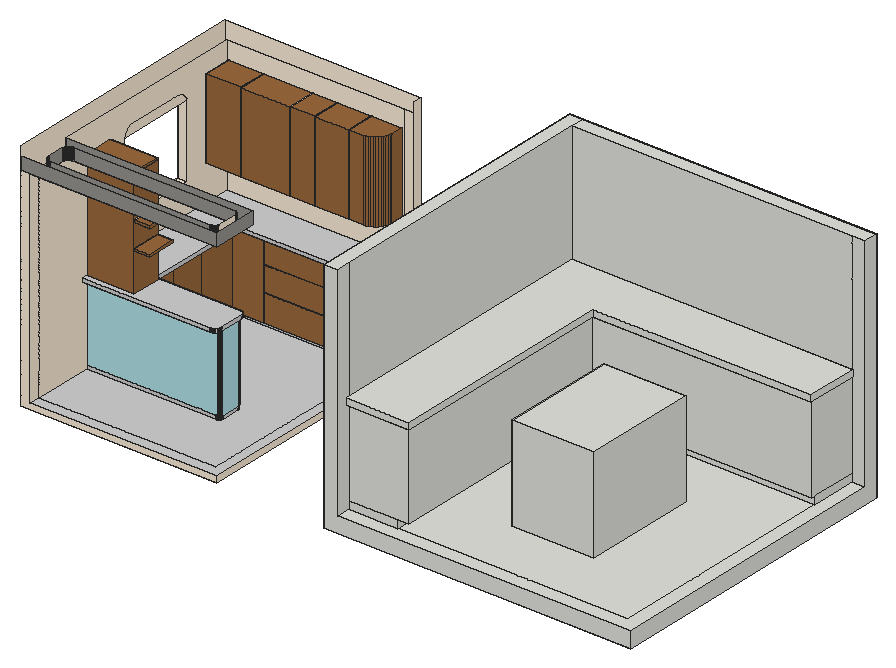
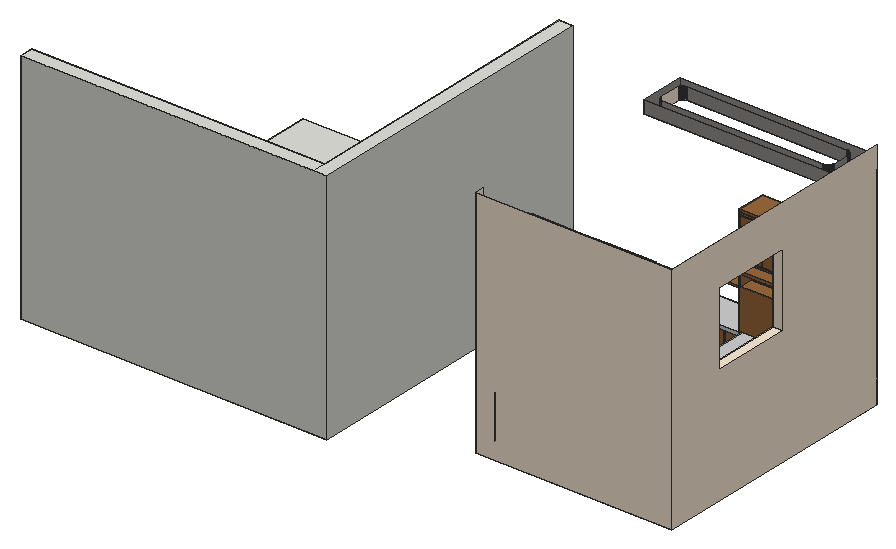
# SketchUp Ruby script. Lengths in inches.
U = 1.inch
M = Sketchup.active_model
def pt(a) = Geom::Point3d.new(a.map { |v| v * U })
def face(e, loops, mat)
  f = e.add_face(loops[0].map { |a| pt(a) })
  loops[1..].each { |l| e.add_face(l.map { |a| pt(a) }).erase! }
  f.material = f.back_material = mat if mat
  f
end
# faces: each face lists its corners as indices into pts; further lists are holes
def faces(e, pts, list, mat = nil) = list.each { |f| face(e, (f[0].is_a?(Array) ? f : [f]).map { |l| l.map { |i| pts[i] } }, mat) }
# xy, xz, yz: faces in a plane at the given z, y or x. An outline is a flat list of corners, or four numbers for a rectangle; further outlines are holes
def ring(l) = l.size == 4 ? [[l[0], l[1]], [l[2], l[1]], [l[2], l[3]], [l[0], l[3]]] : l.each_slice(2).to_a
def flat(e, list, mat, &to3) = list.each { |f| face(e, (f[0].is_a?(Array) ? f : [f]).map { |l| ring(l).map { |u, v| to3.(u, v) } }, mat) }
def xy(e, z, list, mat = nil) = flat(e, list, mat) { |x, y| [x, y, z] }
def xz(e, y, list, mat = nil) = flat(e, list, mat) { |x, z| [x, y, z] }
def yz(e, x, list, mat = nil) = flat(e, list, mat) { |y, z| [x, y, z] }
def lines(e, pts, list) = list.each { |a, b| e.add_line(pt(pts[a]), pt(pts[b])) }
# prism: a flat outline (further loops are holes) pulled along v
def prism(e, loops, v, mat = nil)
  f = face(e, loops, mat); d = Geom::Vector3d.new(v.map { |x| x * U })
  f.pushpull(f.normal.samedirection?(d) ? d.length : -d.length)
end
def box(e, o, s, mat = nil) = prism(e, [[o, [o[0] + s[0], o[1], o[2]], [o[0] + s[0], o[1] + s[1], o[2]], [o[0], o[1] + s[1], o[2]]]], [0, 0, s[2]], mat)
def at(x, y, z, deg = 0) = Geom::Transformation.translation(pt([x, y, z])) * Geom::Transformation.rotation(ORIGIN, Z_AXIS, deg.degrees)
def axes(o, x, y, z) = Geom::Transformation.new([*x, 0, *y, 0, *z, 0, *pt(o).to_a, 1])
def part(name) = M.definitions.add(name)
# library, detail: a bought-in or finely detailed component or shape, given as its bounding box
def library(name, o, s) = part(name).tap { |d| box(d.entities, o, s) }
def detail(e, o, s) = box(e.add_group.entities, o, s)
def put(e, d, t, mat = nil) = e.add_instance(d, t).tap { |i| i.material = mat if mat }
def group(e, t, mat = nil) = e.add_group.tap { |g| g.transformation = t; g.material = mat if mat }.entities
root = M.entities
M.materials.add("[0028_AntiqueWhite]").color = [250, 235, 215]
M.materials.add("[0094_PowderBlue]").color = [176, 224, 230]
M.materials.add("[0095_LightBlue]").color = [173, 216, 230]
M.materials.add("[Carrera Marble]").color = [207, 207, 207]
M.materials.add("[Granite Light Gray]").color = [149, 148, 144]
M.materials.add("[Wood Floor]").color = [155, 105, 61]
xy(root,0,[[313.34,0,630.34,317]])
xy(root,3.27,[[0,0,203.125,263.6875]],"[0028_AntiqueWhite]")
xy(root,9.21,[[10.23,0,203.125,0,203.125,253.46,188.43,253.46,189.04,253.33,189.625,253.14,190.1875,252.87,190.71,252.54,191.19,252.15,191.625,251.71,192,251.22,192.32,250.6875,192.57,250.12,192.75,249.53,192.86,248.92,192.89,248.3,192.89,11.5625,10.23,11.5625],[10.23,11.5625,192.89,11.5625,192.89,223.31,192.85,222.61,192.71,221.92,192.49,221.26,192.18,220.63,191.79,220.05,191.32,219.52,190.8,219.06,190.21,218.67,189.59,218.36,188.92,218.13,188.23,218,187.53,217.95,44.21,217.95,44.21,99.7,144.02,99.7,144.6,99.66,145.16,99.55,145.7,99.37,146.21,99.11,146.6875,98.8,147.12,98.42,147.49,97.99,147.8125,97.51,148.07,97,148.25,96.46,148.36,95.9,148.4,95.33,148.4,76.65,148.29,76.11,148.11,75.59,147.875,75.09,147.58,74.63,147.23,74.2,146.84,73.82,146.4,73.49,145.93,73.21,145.43,72.99,144.91,72.83,144.37,72.73,143.82,72.7,10.23,72.7]],"[Carrera Marble]")
xy(root,13.4,[[44.71,99.7,44.71,101.2,47.02,101.2,47.02,102.89,74.24,102.89,74.24,99.7],[74.74,99.7,110.3,102.89],[110.8,99.7,144.3,102.89],[44.21,101.2,44.21,138.64,47.02,138.64,47.02,102.89,44.71,102.89,44.71,101.2],[44.71,101.2,47.02,102.89],
  [44.21,139.14,47.02,174.76],[44.21,175.26,44.21,216.45,45.71,216.45,45.71,214.45,47.02,214.45,47.02,175.26],[45.71,214.45,47.02,216.45],[47.02,214.45,47.02,216.45,45.71,216.45,45.71,217.95,79.77,217.95,79.77,214.45],[80.27,214.45,151.02,217.95],
  [151.52,214.45,187.8,217.95]],"[0028_AntiqueWhite]")
xy(root,16.1875,[[327.62,0,630.34,0,630.34,302.72,616.07,302.72,616.07,14.28,327.62,14.28],[378.34,14.28,616.07,255.04]])
xy(root,23.9375,[[378.34,14.28,378.34,256.85,400.15,256.85,400.15,251.16,389.53,251.16,389.53,14.28],[400.15,251.16,400.15,256.85,378.34,256.85,378.34,302.72,616.07,302.72,616.07,251.16]])
xy(root,41.65,[[80.27,214.45,151.02,217.95]],"[0028_AntiqueWhite]")
xy(root,42.15,[[80.27,214.45,151.02,217.95]],"[0028_AntiqueWhite]")
xy(root,67.84,[[80.27,214.45,151.02,217.95]],"[Wood Floor]")
xy(root,68.34,[[80.27,214.45,151.02,217.95]],"[Wood Floor]")
xy(root,91.52,[[44.71,99.7,74.24,99.7,74.24,102.89,47.02,102.89,47.02,101.2,44.71,101.2],[74.74,99.7,110.3,102.89],[110.8,99.7,144.3,102.89],[44.21,101.2,44.71,101.2,44.71,102.89,47.02,102.89,47.02,138.64,44.21,138.64],[44.71,101.2,47.02,102.89],
  [44.21,139.14,47.02,174.76],[44.21,175.26,47.02,175.26,47.02,214.45,45.71,214.45,45.71,216.45,44.21,216.45],[45.71,214.45,47.02,216.45],[47.02,214.45,79.77,214.45,79.77,217.95,45.71,217.95,45.71,216.45,47.02,216.45],[80.27,214.45,151.02,217.95],
  [151.52,214.45,187.8,217.95]],"[0028_AntiqueWhite]")
xy(root,92.02,[[10.23,67.2,10.23,253.46,192.89,253.46,192.89,221.5,192.8125,220.24,192.5625,219,192.16,217.8,191.6,216.66,190.89,215.61,190.06,214.66,189.11,213.82,188.06,213.12,186.92,212.5625,185.72,212.15,184.48,211.91,183.22,211.82,56.15,211.82,56.15,105.01,142.61,105.01,143.36,104.97,144.11,104.83,144.83,104.61,145.53,104.31,146.18,103.92,146.78,103.47,147.32,102.9375,147.8,102.35,148.21,101.71,148.53,101.03,148.78,100.3125,148.93,99.57,148.93,74.1875,148.875,73.27,148.7,72.38,148.4,71.51,148,70.69,147.49,69.93,146.89,69.25,146.2,68.64,145.44,68.14,144.62,67.73,143.75,67.4375,142.86,67.26,141.95,67.2]],"[0028_AntiqueWhite]")
xy(root,95.52,[[10.23,67.2,141.95,67.2,142.86,67.26,143.75,67.4375,144.62,67.73,145.44,68.14,146.2,68.64,146.89,69.25,147.49,69.93,148,70.69,148.4,71.51,148.7,72.38,148.875,73.27,148.93,74.1875,148.93,99.57,148.78,100.3125,148.53,101.03,148.21,101.71,147.8,102.35,147.32,102.9375,146.78,103.47,146.18,103.92,145.53,104.31,144.83,104.61,144.11,104.83,143.36,104.97,142.61,105.01,56.15,105.01,56.15,211.82,183.22,211.82,184.48,211.91,185.72,212.15,186.92,212.5625,188.06,213.12,189.11,213.82,190.06,214.66,190.89,215.61,191.6,216.66,192.16,217.8,192.5625,219,192.8125,220.24,192.89,221.5,192.89,253.46,10.23,253.46,10.23,102.82,59.29,102.82,59.29,72.57,10.23,72.57]],"[Carrera Marble]")
xy(root,114.0625,[[327.62,10.96,392.71,14.28],[389.53,14.28,392.71,248.66],[389.53,248.66,617.63,302.72]])
xy(root,120.6875,[[327.62,10.96,392.71,10.96,392.71,248.66,617.63,248.66,617.63,302.72,327.62,302.72]])
xy(root,124.52,[[0,120.375,10.23,202.75]],"[0028_AntiqueWhite]")
xy(root,133.59,[[12.23,224.21,48.23,253.46],[48.73,224.21,98.92,253.46],[99.42,224.21,124.36,253.46],[124.86,224.21,159.42,253.46],[159.92,224.21,159.92,253.46,190.89,253.46,190.89,241.28,190.8,239.6875,190.76,239.17,190.38,237.11,189.74,235.1,188.87,233.19,187.76,231.39,186.44,229.75,184.9375,228.28,183.26,227.01,181.44,225.95,179.51,225.12,177.48,224.54,175.41,224.21]],"[Wood Floor]")
xy(root,135.54,[[59.29,72.57,75.67,102.82]],"[Wood Floor]")
xy(root,137.54,[[59.29,72.57,75.67,102.82],[12.23,89.76,57.29,102.82]],"[Wood Floor]")
xy(root,148.79,[[12.23,89.76,57.29,102.82]],"[Wood Floor]")
xy(root,150.79,[[12.23,89.76,57.29,102.82]],"[Wood Floor]")
xy(root,161.85,[[59.29,72.57,75.67,102.82],[12.23,89.76,57.29,102.82]],"[Wood Floor]")
xy(root,163.85,[[59.29,72.57,75.67,102.82]],"[Wood Floor]")
xy(root,164.15,[[12.23,102.82,34.61,104.76],[34.81,102.82,57.29,104.76]],"[Wood Floor]")
xy(root,200.46,[[0,120.375,10.23,202.75]],"[0028_AntiqueWhite]")
xy(root,203.84,[[12.23,102.82,34.61,104.76],[34.81,102.82,57.29,104.76]],"[Wood Floor]")
xy(root,205.84,[[10.23,72.26,59.67,72.57],[59.29,72.57,59.67,103.14],[10.23,102.82,59.29,103.14]],"[0028_AntiqueWhite]")
xy(root,206.27,[[10.23,72.26,59.67,72.57],[59.29,72.57,59.67,103.14],[10.23,102.82,59.29,103.14]],"[Wood Floor]")
xy(root,208.27,[[10.23,72.57,59.29,102.82]],"[Wood Floor]")
xy(root,216.15,[[12.23,224.21,48.23,253.46],[48.73,224.21,98.92,253.46],[99.42,224.21,124.36,253.46],[124.86,224.21,159.42,253.46],[159.92,224.21,175.41,224.21,177.48,224.54,179.51,225.12,181.44,225.95,183.26,227.01,184.9375,228.28,186.44,229.75,187.76,231.39,188.87,233.19,189.74,235.1,190.38,237.11,190.76,239.17,190.89,241.28,190.89,253.46,159.92,253.46]],"[Wood Floor]")
xy(root,221.34,[[[10.23,0,203.125,45.92],[24.97,7.66,190.05,7.66,190.7,7.7,191.34,7.8125,191.97,8,192.5625,8.27,193.125,8.6,193.64,9,194.11,9.46,194.52,9.97,194.86,10.52,195.14,11.11,195.34,11.73,195.47,12.37,195.47,33.28,195.35,33.9,195.16,34.5,194.92,35.08,194.61,35.63,194.24,36.14,193.82,36.61,193.35,37.03,192.84,37.4,192.29,37.71,191.71,37.96,191.11,38.14,190.49,38.26,24.48,38.26,23.62,38.21,22.77,38.04,21.95,37.76,21.18,37.38,20.47,36.9,19.82,36.33,19.25,35.69,18.77,34.97,18.39,34.2,18.11,33.38,17.94,32.53,17.89,31.67,17.89,14.74,17.95,13.82,18.13,12.91,18.43,12.03,18.84,11.2,19.35,10.43,19.96,9.73,20.66,9.12,21.43,8.61,22.26,8.2,23.14,7.9,24.05,7.72]]],"[Granite Light Gray]")
xy(root,243.9,[[313.34,0,327.62,317],[327.62,302.72,630.34,317]])
xz(root,0,[[313.34,0,630.34,0,630.34,16.1875,327.62,16.1875,327.62,243.9,313.34,243.9]])
xz(root,0,[[0,3.27,203.125,3.27,203.125,9.21,10.23,9.21,10.23,221.34,0,221.34]],"[0028_AntiqueWhite]")
xz(root,0,[[0,221.34,203.125,234.21]],"[Granite Light Gray]")
xz(root,7.66,[[24.97,221.34,190.05,233.77]],"[Granite Light Gray]")
xz(root,10.96,[[327.62,114.0625,392.71,120.6875]])
xz(root,38.26,[[24.48,221.34,190.49,233.77]],"[Granite Light Gray]")
xz(root,45.92,[[10.23,221.34,203.125,234.21]],"[Granite Light Gray]")
xz(root,67.2,[[10.23,92.02,141.95,95.52]],"[Carrera Marble]")
xz(root,72.26,[[10.23,205.84,59.67,206.27]],"[Wood Floor]")
xz(root,72.57,[[10.23,95.52,59.29,205.84],[59.29,135.54,75.67,137.54],[59.29,161.85,75.67,163.85],[10.23,206.27,59.29,208.27]],"[Wood Floor]")
xz(root,89.76,[[12.23,137.54,57.29,148.79],[12.23,150.79,57.29,161.85]],"[Wood Floor]")
xz(root,99.7,[[44.21,9.21,144.02,12.9],[44.71,13.4,74.24,91.52],[74.74,13.4,110.3,91.52],[110.8,13.4,144.3,91.52]],"[0028_AntiqueWhite]")
xz(root,101.2,[[44.21,13.4,47.02,91.52]],"[0028_AntiqueWhite]")
xz(root,102.82,[[[10.23,95.52,59.29,205.84],[34.81,164.15,57.29,203.84],[12.23,164.15,34.61,203.84],[12.23,137.54,57.29,148.79],[12.23,150.79,57.29,161.85]],[59.29,135.54,75.67,137.54],[59.29,161.85,75.67,163.85],[10.23,206.27,59.29,208.27]],"[Wood Floor]")
xz(root,102.89,[[44.71,13.4,74.24,91.52],[74.74,13.4,110.3,91.52],[110.8,13.4,144.3,91.52]],"[Wood Floor]")
xz(root,103.14,[[10.23,205.84,59.67,206.27]],"[Wood Floor]")
xz(root,104.76,[[12.23,164.15,34.61,203.84],[34.81,164.15,57.29,203.84]],"[Wood Floor]")
xz(root,105.01,[[56.15,92.02,142.61,95.52]],"[Carrera Marble]")
xz(root,120.375,[[0,124.52,10.23,200.46]],"[0028_AntiqueWhite]")
xz(root,138.64,[[44.21,13.4,47.02,91.52]],"[Wood Floor]")
xz(root,139.14,[[44.21,13.4,47.02,91.52]],"[Wood Floor]")
xz(root,174.76,[[44.21,13.4,47.02,91.52]],"[Wood Floor]")
xz(root,175.26,[[44.21,13.4,47.02,91.52]],"[Wood Floor]")
xz(root,202.75,[[0,124.52,10.23,200.46]],"[0028_AntiqueWhite]")
xz(root,211.82,[[56.15,92.02,183.22,95.52]],"[Carrera Marble]")
xz(root,214.45,[[45.71,13.4,79.77,91.52],[80.27,13.4,151.02,41.65],[151.52,13.4,187.8,91.52],[80.27,42.15,151.02,67.84],[80.27,68.34,151.02,91.52]],"[Wood Floor]")
xz(root,216.45,[[44.21,13.4,47.02,91.52]],"[0028_AntiqueWhite]")
xz(root,217.95,[[45.71,13.4,79.77,91.52],[80.27,13.4,151.02,41.65],[151.52,13.4,187.8,91.52],[80.27,42.15,151.02,67.84],[80.27,68.34,151.02,91.52]],"[0028_AntiqueWhite]")
xz(root,224.21,[[12.23,133.59,48.23,216.15],[48.73,133.59,98.92,216.15],[99.42,133.59,124.36,216.15],[124.86,133.59,159.42,216.15],[159.92,133.59,175.41,216.15]],"[Wood Floor]")
xz(root,248.66,[[392.71,114.0625,617.63,120.6875]])
xz(root,253.46,[[188.43,9.21,192.89,12.9],[192.89,9.21,203.125,234.21],[189.47,12.9,192.89,92.02],[[10.23,95.52,192.89,234.21],[48.73,133.59,98.92,216.15],[12.23,133.59,48.23,216.15],[124.86,133.59,159.42,216.15],[159.92,133.59,190.89,216.15],[99.42,133.59,124.36,216.15]]],"[0028_AntiqueWhite]")
xz(root,263.6875,[[0,3.27,203.125,243.9]],"[0028_AntiqueWhite]")
xz(root,302.72,[[616.07,16.1875,630.34,16.1875,630.34,243.9,616.07,243.9,616.07,120.6875,617.63,120.6875,617.63,114.0625,616.07,114.0625],[327.62,120.6875,616.07,243.9]])
xz(root,317,[[313.34,0,630.34,243.9]])
yz(root,0,[[[0,3.27,263.6875,243.9],[120.375,124.52,202.75,200.46]]],"[0028_AntiqueWhite]")
yz(root,10.23,[[0,9.21,11.5625,221.34],[[11.5625,9.21,72.7,9.21,72.7,92.02,67.2,92.02,67.2,95.52,72.57,95.52,72.57,205.84,72.26,205.84,72.26,206.27,72.57,206.27,72.57,208.27,102.82,208.27,102.82,206.27,103.14,206.27,103.14,205.84,102.82,205.84,102.82,95.52,253.46,95.52,253.46,234.21,45.92,234.21,45.92,221.34,11.5625,221.34],[120.375,124.52,120.375,200.46,120.84,201.84,121.46,203.17,122.21,204.42,123.09,205.58,124.1,206.64,125.21,207.59,126.42,208.41,127.71,209.09,129.07,209.63,130.47,210.02,131.92,210.26,133.375,210.34,189.75,210.34,191.21,210.26,192.65,210.02,194.06,209.63,195.41,209.09,196.7,208.41,197.91,207.59,199.03,206.64,200.03,205.58,200.91,204.42,201.67,203.17,202.28,201.84,202.75,200.46,202.75,124.52]],[120.375,200.46,202.75,200.46,202.28,201.84,201.67,203.17,200.91,204.42,200.03,205.58,199.03,206.64,197.91,207.59,196.7,208.41,195.41,209.09,194.06,209.63,192.65,210.02,191.21,210.26,189.75,210.34,133.375,210.34,131.92,210.26,130.47,210.02,129.07,209.63,127.71,209.09,126.42,208.41,125.21,207.59,124.1,206.64,123.09,205.58,122.21,204.42,121.46,203.17,120.84,201.84]],"[0028_AntiqueWhite]")
yz(root,12.23,[[102.82,164.15,104.76,203.84]],"[0028_AntiqueWhite]")
yz(root,12.23,[[224.21,133.59,253.46,216.15],[89.76,137.54,102.82,148.79],[89.76,150.79,102.82,161.85]],"[Wood Floor]")
yz(root,17.89,[[14.74,221.34,31.67,233.77]],"[Granite Light Gray]")
yz(root,34.61,[[102.82,164.15,104.76,203.84]],"[Wood Floor]")
yz(root,34.81,[[102.82,164.15,104.76,203.84]],"[0028_AntiqueWhite]")
yz(root,44.21,[[101.2,13.4,138.64,91.52],[139.14,13.4,174.76,91.52],[175.26,13.4,216.45,91.52]],"[0028_AntiqueWhite]")
yz(root,44.71,[[99.7,13.4,102.89,91.52]],"[0028_AntiqueWhite]")
yz(root,45.71,[[214.45,13.4,217.95,91.52]],"[0028_AntiqueWhite]")
yz(root,47.02,[[101.2,13.4,138.64,91.52],[139.14,13.4,174.76,91.52],[175.26,13.4,216.45,91.52]],"[Wood Floor]")
yz(root,48.23,[[224.21,133.59,253.46,216.15]],"[0028_AntiqueWhite]")
yz(root,48.73,[[224.21,133.59,253.46,216.15]],"[0028_AntiqueWhite]")
yz(root,56.15,[[105.01,92.02,211.82,95.52]],"[Carrera Marble]")
yz(root,57.29,[[89.76,137.54,102.82,148.79],[89.76,150.79,102.82,161.85],[102.82,164.15,104.76,203.84]],"[Wood Floor]")
yz(root,59.29,[[72.57,135.54,102.82,137.54],[72.57,161.85,102.82,163.85]],"[0028_AntiqueWhite]")
yz(root,59.29,[[72.57,95.52,102.82,135.54],[72.57,137.54,102.82,161.85],[72.57,163.85,102.82,205.84],[72.57,206.27,102.82,208.27]],"[Wood Floor]")
yz(root,59.67,[[72.26,205.84,103.14,206.27]],"[Wood Floor]")
yz(root,74.24,[[99.7,13.4,102.89,91.52]],"[0028_AntiqueWhite]")
yz(root,74.74,[[99.7,13.4,102.89,91.52]],"[0028_AntiqueWhite]")
yz(root,75.67,[[72.57,135.54,102.82,137.54],[72.57,161.85,102.82,163.85]],"[Wood Floor]")
yz(root,79.77,[[214.45,13.4,217.95,91.52]],"[0028_AntiqueWhite]")
yz(root,80.27,[[214.45,13.4,217.95,41.65],[214.45,42.15,217.95,67.84],[214.45,68.34,217.95,91.52]],"[0028_AntiqueWhite]")
yz(root,98.92,[[224.21,133.59,253.46,216.15]],"[0028_AntiqueWhite]")
yz(root,99.42,[[224.21,133.59,253.46,216.15]],"[0028_AntiqueWhite]")
yz(root,110.3,[[99.7,13.4,102.89,91.52]],"[0028_AntiqueWhite]")
yz(root,110.8,[[99.7,13.4,102.89,91.52]],"[0028_AntiqueWhite]")
yz(root,124.36,[[224.21,133.59,253.46,216.15]],"[0028_AntiqueWhite]")
yz(root,124.86,[[224.21,133.59,253.46,216.15]],"[0028_AntiqueWhite]")
yz(root,144.3,[[99.7,13.4,102.89,91.52]],"[Wood Floor]")
yz(root,148.93,[[74.1875,92.02,99.57,95.52]],"[Carrera Marble]")
yz(root,151.02,[[214.45,13.4,217.95,41.65]],"[0028_AntiqueWhite]")
yz(root,151.02,[[214.45,42.15,217.95,67.84],[214.45,68.34,217.95,91.52]],"[Wood Floor]")
yz(root,151.52,[[214.45,13.4,217.95,91.52]],"[0028_AntiqueWhite]")
yz(root,159.42,[[224.21,133.59,253.46,216.15]],"[0028_AntiqueWhite]")
yz(root,159.92,[[224.21,133.59,253.46,216.15]],"[0028_AntiqueWhite]")
yz(root,187.8,[[214.45,13.4,217.95,91.52]],"[Wood Floor]")
yz(root,190.89,[[241.28,133.59,253.46,216.15]],"[Wood Floor]")
yz(root,192.89,[[221.5,92.02,253.46,95.52]],"[Carrera Marble]")
yz(root,195.47,[[12.37,221.34,33.28,233.77]],"[0028_AntiqueWhite]")
yz(root,203.125,[[0,3.27,263.6875,3.27,263.6875,243.9,253.46,243.9,253.46,9.21,0,9.21]],"[0028_AntiqueWhite]")
yz(root,203.125,[[0,221.34,45.92,234.21]],"[Granite Light Gray]")
yz(root,313.34,[[0,0,317,243.9]])
yz(root,327.62,[[0,16.1875,14.28,16.1875,14.28,114.0625,10.96,114.0625,10.96,120.6875,14.28,120.6875,14.28,243.9,0,243.9],[14.28,120.6875,302.72,243.9]])
yz(root,392.71,[[10.96,114.0625,248.66,120.6875]])
yz(root,617.63,[[248.66,114.0625,302.72,120.6875]])
yz(root,630.34,[[0,0,317,0,317,243.9,302.72,243.9,302.72,16.1875,0,16.1875]])
p = [[142.86,67.26,95.52],[141.95,67.2,95.52],[141.95,67.2,92.02],[142.86,67.26,92.02],[143.75,67.4375,95.52],[143.75,67.4375,92.02],
  [144.62,67.73,95.52],[144.62,67.73,92.02],[145.44,68.14,95.52],[145.44,68.14,92.02],[146.2,68.64,95.52],[146.2,68.64,92.02],
  [146.89,69.25,95.52],[146.89,69.25,92.02],[147.49,69.93,95.52],[147.49,69.93,92.02],[148,70.69,95.52],[148,70.69,92.02],
  [148.4,71.51,95.52],[148.4,71.51,92.02],[148.7,72.38,95.52],[148.7,72.38,92.02],[148.875,73.27,95.52],[148.875,73.27,92.02],
  [148.93,74.1875,95.52],[148.93,74.1875,92.02],[148.78,100.3125,95.52],[148.93,99.57,95.52],[148.93,99.57,92.02],[148.78,100.3125,92.02],
  [148.53,101.03,95.52],[148.53,101.03,92.02],[148.21,101.71,95.52],[148.21,101.71,92.02],[147.8,102.35,95.52],[147.8,102.35,92.02],
  [147.32,102.9375,95.52],[147.32,102.9375,92.02],[146.78,103.47,95.52],[146.78,103.47,92.02],[146.18,103.92,95.52],[146.18,103.92,92.02],
  [145.53,104.31,95.52],[145.53,104.31,92.02],[144.83,104.61,95.52],[144.83,104.61,92.02],[144.11,104.83,95.52],[144.11,104.83,92.02],
  [143.36,104.97,95.52],[143.36,104.97,92.02],[142.61,105.01,95.52],[142.61,105.01,92.02],[184.48,211.91,95.52],[183.22,211.82,95.52],
  [183.22,211.82,92.02],[184.48,211.91,92.02],[185.72,212.15,95.52],[185.72,212.15,92.02],[186.92,212.5625,95.52],[186.92,212.5625,92.02],
  [188.06,213.12,95.52],[188.06,213.12,92.02],[189.11,213.82,95.52],[189.11,213.82,92.02],[190.06,214.66,95.52],[190.06,214.66,92.02],
  [190.89,215.61,95.52],[190.89,215.61,92.02],[191.6,216.66,95.52],[191.6,216.66,92.02],[192.16,217.8,95.52],[192.16,217.8,92.02],
  [192.5625,219,95.52],[192.5625,219,92.02],[192.8125,220.24,95.52],[192.8125,220.24,92.02],[192.89,221.5,95.52],[192.89,221.5,92.02],
  [177.48,224.54,216.15],[175.41,224.21,216.15],[175.41,224.21,133.59],[177.48,224.54,133.59],[179.51,225.12,216.15],[179.51,225.12,133.59],
  [181.44,225.95,216.15],[181.44,225.95,133.59],[183.26,227.01,216.15],[183.26,227.01,133.59],[184.9375,228.28,216.15],[184.9375,228.28,133.59],
  [186.44,229.75,216.15],[186.44,229.75,133.59],[187.76,231.39,216.15],[187.76,231.39,133.59],[188.87,233.19,216.15],[188.87,233.19,133.59],
  [189.74,235.1,216.15],[189.74,235.1,133.59],[190.38,237.11,216.15],[190.38,237.11,133.59],[190.76,239.17,216.15],[190.76,239.17,133.59],
  [190.89,241.28,216.15],[190.8,239.6875,133.59],[190.89,241.28,133.59],[24.05,7.72,221.34],[23.14,7.9,221.34],[23.14,7.9,233.77],
  [24.05,7.72,233.77],[24.97,7.66,221.34],[24.97,7.66,233.77],[190.7,7.7,221.34],[190.05,7.66,221.34],[190.05,7.66,233.77],
  [190.7,7.7,233.77],[191.34,7.8125,221.34],[191.34,7.8125,233.77],[191.97,8,221.34],[191.97,8,233.77],[22.26,8.2,221.34],
  [22.26,8.2,233.77],[192.5625,8.27,221.34],[192.5625,8.27,233.77],[21.43,8.61,221.34],[21.43,8.61,233.77],[193.125,8.6,221.34],
  [193.125,8.6,233.77],[20.66,9.12,221.34],[20.66,9.12,233.77],[193.64,9,221.34],[193.64,9,233.77],[194.11,9.46,221.34],
  [194.11,9.46,233.77],[19.96,9.73,221.34],[19.96,9.73,233.77],[194.52,9.97,221.34],[194.52,9.97,233.77],[19.35,10.43,221.34],
  [19.35,10.43,233.77],[194.86,10.52,221.34],[194.86,10.52,233.77],[18.84,11.2,221.34],[18.84,11.2,233.77],[195.14,11.11,221.34],
  [195.14,11.11,233.77],[195.34,11.73,221.34],[195.34,11.73,233.77],[18.43,12.03,221.34],[18.43,12.03,233.77],[195.47,12.37,221.34],
  [195.47,12.37,233.77],[18.13,12.91,221.34],[18.13,12.91,233.77],[17.95,13.82,221.34],[17.95,13.82,233.77],[17.89,14.74,221.34],
  [17.89,14.74,233.77],[17.89,31.67,221.34],[17.94,32.53,221.34],[17.94,32.53,233.77],[17.89,31.67,233.77],[18.11,33.38,221.34],
  [18.11,33.38,233.77],[195.35,33.9,221.34],[195.47,33.28,221.34],[195.47,33.28,233.77],[195.35,33.9,233.77],[18.39,34.2,221.34],
  [18.39,34.2,233.77],[195.16,34.5,221.34],[195.16,34.5,233.77],[18.77,34.97,221.34],[18.77,34.97,233.77],[194.92,35.08,221.34],
  [194.92,35.08,233.77],[19.25,35.69,221.34],[19.25,35.69,233.77],[194.61,35.63,221.34],[194.61,35.63,233.77],[194.24,36.14,221.34],
  [194.24,36.14,233.77],[19.82,36.33,221.34],[19.82,36.33,233.77],[193.82,36.61,221.34],[193.82,36.61,233.77],[20.47,36.9,221.34],
  [20.47,36.9,233.77],[193.35,37.03,221.34],[193.35,37.03,233.77],[21.18,37.38,221.34],[21.18,37.38,233.77],[192.84,37.4,221.34],
  [192.84,37.4,233.77],[21.95,37.76,221.34],[21.95,37.76,233.77],[192.29,37.71,221.34],[192.29,37.71,233.77],[191.71,37.96,221.34],
  [191.71,37.96,233.77],[22.77,38.04,221.34],[22.77,38.04,233.77],[23.62,38.21,221.34],[23.62,38.21,233.77],[191.11,38.14,221.34],
  [191.11,38.14,233.77],[190.49,38.26,221.34],[190.49,38.26,233.77],[24.48,38.26,221.34],[24.48,38.26,233.77]]
faces(root,p,[[0,1,2,3],[4,0,3,5],[6,4,5,7],[8,6,7,9],[10,8,9,11],[12,10,11,13],[14,12,13,15],[16,14,15,17],
  [18,16,17,19],[20,18,19,21],[22,20,21,23],[24,22,23,25],[26,27,28,29],[30,26,29,31],[32,30,31,33],[34,32,33,35],
  [36,34,35,37],[38,36,37,39],[40,38,39,41],[42,40,41,43],[44,42,43,45],[46,44,45,47],[48,46,47,49],[50,48,49,51],
  [52,53,54,55],[56,52,55,57],[58,56,57,59],[60,58,59,61],[62,60,61,63],[64,62,63,65],[66,64,65,67],[68,66,67,69],
  [70,68,69,71],[72,70,71,73],[74,72,73,75],[76,74,75,77]],"[Carrera Marble]")
faces(root,p,[[78,79,80,81],[82,78,81,83],[84,82,83,85],[86,84,85,87],[88,86,87,89],[90,88,89,91],[92,90,91,93],[94,92,93,95],
  [96,94,95,97],[98,96,97,99],[100,98,99,101],[102,100,101,103,104]],"[Wood Floor]")
faces(root,p,[[105,106,107,108],[109,105,108,110],[106,119,120,107],[119,123,124,120],[123,127,128,124],[127,133,134,128],[133,137,138,134],[137,141,142,138],
  [141,147,148,142],[147,151,152,148],[151,153,154,152],[153,155,156,154],[157,158,159,160],[158,161,162,159],[161,167,168,162],[167,171,172,168],
  [171,175,176,172],[175,181,182,176],[181,185,186,182],[185,189,190,186],[189,193,194,190],[193,199,200,194],[199,201,202,200],[201,207,208,202]],"[Granite Light Gray]")
faces(root,p,[[111,112,113,114],[115,111,114,116],[117,115,116,118],[121,117,118,122],[125,121,122,126],[129,125,126,130],[131,129,130,132],[135,131,132,136],
  [139,135,136,140],[143,139,140,144],[145,143,144,146],[149,145,146,150],[163,164,165,166],[169,163,166,170],[173,169,170,174],[177,173,174,178],
  [179,177,178,180],[183,179,180,184],[187,183,184,188],[191,187,188,192],[195,191,192,196],[197,195,196,198],[203,197,198,204],[205,203,204,206]],"[0028_AntiqueWhite]")
g1 = group(root,at(10.23,72.7,9.21),"[0028_AntiqueWhite]")
xy(g1,3.6875,[[0,0,133.59,0,134.13,0.03,134.67,0.13,135.2,0.29,135.7,0.51,136.17,0.79,136.61,1.12,137,1.5,137.35,1.93,137.64,2.39,137.88,2.89,138.05,3.41,138.17,3.95,138.17,22.625,138.13,23.2,138.02,23.76,137.83,24.3,137.58,24.8125,137.26,25.29,136.89,25.72,136.46,26.1,135.98,26.41,135.47,26.67,134.93,26.85,134.36,26.96,133.79,27,33.98,27,33.98,145.25,177.3,145.25,178,145.3,178.69,145.43,179.35,145.66,179.98,145.97,180.57,146.36,181.09,146.82,181.55,147.35,181.94,147.93,182.25,148.56,182.48,149.22,182.62,149.91,182.66,150.61,182.66,175.6,182.625,176.22,182.52,176.83,182.33,177.42,182.08,177.99,181.77,178.52,181.39,179.01,180.96,179.45,180.48,179.84,179.95,180.17,179.39,180.4375,178.81,180.63,178.2,180.76,0,180.76]])
xz(g1,0,[[0,0,133.59,3.6875]],"[Carrera Marble]")
xz(g1,145.25,[[33.98,0,177.3,3.6875]],"[Carrera Marble]")
yz(g1,33.98,[[27,0,145.25,3.6875]],"[Carrera Marble]")
yz(g1,138.17,[[3.95,0,22.625,3.6875]],"[Carrera Marble]")
yz(g1,182.66,[[150.61,0,175.6,3.6875]],"[Carrera Marble]")
p = [[134.13,0.03,3.6875],[133.59,0,3.6875],[133.59,0,0],[134.13,0.03,0],[134.67,0.13,3.6875],[134.67,0.13,0],
  [135.2,0.29,3.6875],[135.2,0.29,0],[135.7,0.51,3.6875],[135.7,0.51,0],[136.17,0.79,3.6875],[136.17,0.79,0],
  [136.61,1.12,3.6875],[136.61,1.12,0],[137,1.5,3.6875],[137,1.5,0],[137.35,1.93,3.6875],[137.35,1.93,0],
  [137.64,2.39,3.6875],[137.64,2.39,0],[137.88,2.89,3.6875],[137.88,2.89,0],[138.05,3.41,3.6875],[138.05,3.41,0],
  [138.17,3.95,3.6875],[138.17,3.95,0],[138.13,23.2,3.6875],[138.17,22.625,3.6875],[138.17,22.625,0],[138.13,23.2,0],
  [138.02,23.76,3.6875],[138.02,23.76,0],[137.83,24.3,3.6875],[137.83,24.3,0],[137.58,24.8125,3.6875],[137.58,24.8125,0],
  [137.26,25.29,3.6875],[137.26,25.29,0],[136.89,25.72,3.6875],[136.89,25.72,0],[136.46,26.1,3.6875],[136.46,26.1,0],
  [135.98,26.41,3.6875],[135.98,26.41,0],[135.47,26.67,3.6875],[135.47,26.67,0],[134.93,26.85,3.6875],[134.93,26.85,0],
  [134.36,26.96,3.6875],[134.36,26.96,0],[133.79,27,3.6875],[133.79,27,0],[178,145.3,3.6875],[177.3,145.25,3.6875],
  [177.3,145.25,0],[178,145.3,0],[178.69,145.43,3.6875],[178.69,145.43,0],[179.35,145.66,3.6875],[179.35,145.66,0],
  [179.98,145.97,3.6875],[179.98,145.97,0],[180.57,146.36,3.6875],[180.57,146.36,0],[181.09,146.82,3.6875],[181.09,146.82,0],
  [181.55,147.35,3.6875],[181.55,147.35,0],[181.94,147.93,3.6875],[181.94,147.93,0],[182.25,148.56,3.6875],[182.25,148.56,0],
  [182.48,149.22,3.6875],[182.48,149.22,0],[182.62,149.91,3.6875],[182.62,149.91,0],[182.66,150.61,3.6875],[182.66,150.61,0],
  [182.625,176.22,3.6875],[182.66,175.6,3.6875],[182.66,175.6,0],[182.625,176.22,0],[182.52,176.83,3.6875],[182.52,176.83,0],
  [182.33,177.42,3.6875],[182.33,177.42,0],[182.08,177.99,3.6875],[182.08,177.99,0],[181.77,178.52,3.6875],[181.77,178.52,0],
  [181.39,179.01,3.6875],[181.39,179.01,0],[180.96,179.45,3.6875],[180.96,179.45,0],[180.48,179.84,3.6875],[180.48,179.84,0],
  [179.95,180.17,3.6875],[179.95,180.17,0],[179.39,180.4375,3.6875],[179.39,180.4375,0],[178.81,180.63,3.6875],[178.81,180.63,0],
  [178.2,180.76,3.6875],[178.2,180.76,0]]
faces(g1,p,[[0,1,2,3],[4,0,3,5],[6,4,5,7],[8,6,7,9],[10,8,9,11],[12,10,11,13],[14,12,13,15],[16,14,15,17],
  [18,16,17,19],[20,18,19,21],[22,20,21,23],[24,22,23,25],[26,27,28,29],[30,26,29,31],[32,30,31,33],[34,32,33,35],
  [36,34,35,37],[38,36,37,39],[40,38,39,41],[42,40,41,43],[44,42,43,45],[46,44,45,47],[48,46,47,49],[50,48,49,51],
  [52,53,54,55],[56,52,55,57],[58,56,57,59],[60,58,59,61],[62,60,61,63],[64,62,63,65],[66,64,65,67],[68,66,67,69],
  [70,68,69,71],[72,70,71,73],[74,72,73,75],[76,74,75,77],[78,79,80,81],[82,78,81,83],[84,82,83,85],[86,84,85,87],
  [88,86,87,89],[90,88,89,91],[92,90,91,93],[94,92,93,95],[96,94,95,97],[98,96,97,99],[100,98,99,101],[102,100,101,103]],"[Carrera Marble]")
g2 = group(root,at(10.23,72.7,12.9),"[0095_LightBlue]")
xy(g2,0,[[0,0,0,180.76,179.24,180.76,179.65,180.64,180.05,180.49,180.42,180.3,180.79,180.07,181.125,179.82,181.4375,179.53,181.72,179.22,181.98,178.88,182.2,178.52,182.39,178.14,182.55,177.74,182.66,177.34,182.66,148.84,182.63,148.37,182.54,147.91,182.39,147.47,182.18,147.04,181.92,146.65,181.61,146.3,181.26,145.99,180.87,145.73,180.45,145.52,180,145.37,179.54,145.28,179.07,145.25,33.98,145.25,33.98,27,134.57,27,135.08,26.97,135.58,26.87,136.07,26.7,136.52,26.48,136.95,26.19,137.34,25.85,137.67,25.47,137.96,25.04,138.18,24.59,138.35,24.1,138.45,23.6,138.48,23.09,138.48,3.3,138.375,2.9,138.23,2.51,138.05,2.14,137.84,1.79,137.6,1.47,137.32,1.16,137.02,0.89,136.6875,0.64,136.34,0.43,135.97,0.25,135.58,0.11,135.1875,0]])
xy(g2,79.125,[[0,0,135.1875,0,135.58,0.11,135.97,0.25,136.34,0.43,136.6875,0.64,137.02,0.89,137.32,1.16,137.6,1.47,137.84,1.79,138.05,2.14,138.23,2.51,138.375,2.9,138.48,3.3,138.48,23.09,138.45,23.6,138.35,24.1,138.18,24.59,137.96,25.04,137.67,25.47,137.34,25.85,136.95,26.19,136.52,26.48,136.07,26.7,135.58,26.87,135.08,26.97,134.57,27,33.98,27,33.98,145.25,179.07,145.25,179.54,145.28,180,145.37,180.45,145.52,180.87,145.73,181.26,145.99,181.61,146.3,181.92,146.65,182.18,147.04,182.39,147.47,182.54,147.91,182.63,148.37,182.66,148.84,182.66,177.34,182.55,177.74,182.39,178.14,182.2,178.52,181.98,178.88,181.72,179.22,181.4375,179.53,181.125,179.82,180.79,180.07,180.42,180.3,180.05,180.49,179.65,180.64,179.24,180.76,0,180.76]])
xz(g2,0,[[0,0,135.1875,79.125]],"[0094_PowderBlue]")
xz(g2,27,[[33.98,0,134.57,79.125]])
xz(g2,145.25,[[33.98,0,179.07,79.125]])
yz(g2,33.98,[[27,0,145.25,79.125]])
yz(g2,138.48,[[3.3,0,23.09,79.125]],"[0094_PowderBlue]")
yz(g2,182.66,[[148.84,0,177.34,79.125]])
p = [[135.58,0.11,79.125],[135.1875,0,79.125],[135.1875,0,0],[135.58,0.11,0],[135.97,0.25,79.125],[135.97,0.25,0],
  [136.34,0.43,79.125],[136.34,0.43,0],[136.6875,0.64,79.125],[136.6875,0.64,0],[137.02,0.89,79.125],[137.02,0.89,0],
  [137.32,1.16,79.125],[137.32,1.16,0],[137.6,1.47,79.125],[137.6,1.47,0],[137.84,1.79,79.125],[137.84,1.79,0],
  [138.05,2.14,79.125],[138.05,2.14,0],[138.23,2.51,79.125],[138.23,2.51,0],[138.375,2.9,79.125],[138.375,2.9,0],
  [138.48,3.3,79.125],[138.48,3.3,0],[138.45,23.6,79.125],[138.48,23.09,79.125],[138.48,23.09,0],[138.45,23.6,0],
  [138.35,24.1,79.125],[138.35,24.1,0],[138.18,24.59,79.125],[138.18,24.59,0],[137.96,25.04,79.125],[137.96,25.04,0],
  [137.67,25.47,79.125],[137.67,25.47,0],[137.34,25.85,79.125],[137.34,25.85,0],[136.95,26.19,79.125],[136.95,26.19,0],
  [136.52,26.48,79.125],[136.52,26.48,0],[136.07,26.7,79.125],[136.07,26.7,0],[135.58,26.87,79.125],[135.58,26.87,0],
  [135.08,26.97,79.125],[135.08,26.97,0],[134.57,27,79.125],[134.57,27,0],[179.54,145.28,79.125],[179.07,145.25,79.125],
  [179.07,145.25,0],[179.54,145.28,0],[180,145.37,79.125],[180,145.37,0],[180.45,145.52,79.125],[180.45,145.52,0],
  [180.87,145.73,79.125],[180.87,145.73,0],[181.26,145.99,79.125],[181.26,145.99,0],[181.61,146.3,79.125],[181.61,146.3,0],
  [181.92,146.65,79.125],[181.92,146.65,0],[182.18,147.04,79.125],[182.18,147.04,0],[182.39,147.47,79.125],[182.39,147.47,0],
  [182.54,147.91,79.125],[182.54,147.91,0],[182.63,148.37,79.125],[182.63,148.37,0],[182.66,148.84,79.125],[182.66,148.84,0],
  [182.55,177.74,79.125],[182.66,177.34,79.125],[182.66,177.34,0],[182.55,177.74,0],[182.39,178.14,79.125],[182.39,178.14,0],
  [182.2,178.52,79.125],[182.2,178.52,0],[181.98,178.88,79.125],[181.98,178.88,0],[181.72,179.22,79.125],[181.72,179.22,0],
  [181.4375,179.53,79.125],[181.4375,179.53,0],[181.125,179.82,79.125],[181.125,179.82,0],[180.79,180.07,79.125],[180.79,180.07,0],
  [180.42,180.3,79.125],[180.42,180.3,0],[180.05,180.49,79.125],[180.05,180.49,0],[179.65,180.64,79.125],[179.65,180.64,0],
  [179.24,180.76,79.125],[179.24,180.76,0]]
faces(g2,p,[[0,1,2,3],[4,0,3,5],[6,4,5,7],[8,6,7,9],[10,8,9,11],[12,10,11,13],[14,12,13,15],[16,14,15,17],
  [18,16,17,19],[20,18,19,21],[22,20,21,23],[24,22,23,25],[26,27,28,29],[30,26,29,31],[32,30,31,33],[34,32,33,35],
  [36,34,35,37],[38,36,37,39],[40,38,39,41],[42,40,41,43],[44,42,43,45],[46,44,45,47],[48,46,47,49],[50,48,49,51]],"[0094_PowderBlue]")
faces(g2,p,[[52,53,54,55],[56,52,55,57],[58,56,57,59],[60,58,59,61],[62,60,61,63],[64,62,63,65],[66,64,65,67],[68,66,67,69],
  [70,68,69,71],[72,70,71,73],[74,72,73,75],[76,74,75,77],[78,79,80,81],[82,78,81,83],[84,82,83,85],[86,84,85,87],
  [88,86,87,89],[90,88,89,91],[92,90,91,93],[94,92,93,95],[96,94,95,97],[98,96,97,99],[100,98,99,101],[102,100,101,103]])
g3 = group(root,at(447.74,74.97,16.1875))
xy(g3,97.875,[[0,0,84.0625,119.125]])
xz(g3,0,[[0,0,84.0625,97.875]])
xz(g3,119.125,[[0,0,84.0625,97.875]])
yz(g3,0,[[0,0,119.125,97.875]])
yz(g3,84.0625,[[0,0,119.125,97.875]])
g4 = group(root,at(327.62,14.28,16.1875))
xy(g4,7.75,[[0,0,50.72,0,50.72,240.76,288.45,240.76,288.45,288.45,0,288.45]])
xz(g4,0,[[0,0,50.72,7.75]])
xz(g4,240.76,[[50.72,0,288.45,7.75]])
yz(g4,50.72,[[0,0,240.76,7.75]])
yz(g4,288.45,[[240.76,0,288.45,7.75]])
g5 = group(root,at(327.62,14.28,23.9375))
xy(g5,90.125,[[0,0,61.91,0,61.91,236.89,288.45,236.89,288.45,288.45,0,288.45]])
xz(g5,0,[[0,0,61.91,90.125]])
xz(g5,236.89,[[61.91,0,288.45,90.125]])
yz(g5,61.91,[[0,0,236.89,90.125]])
yz(g5,288.45,[[236.89,0,288.45,90.125]])
